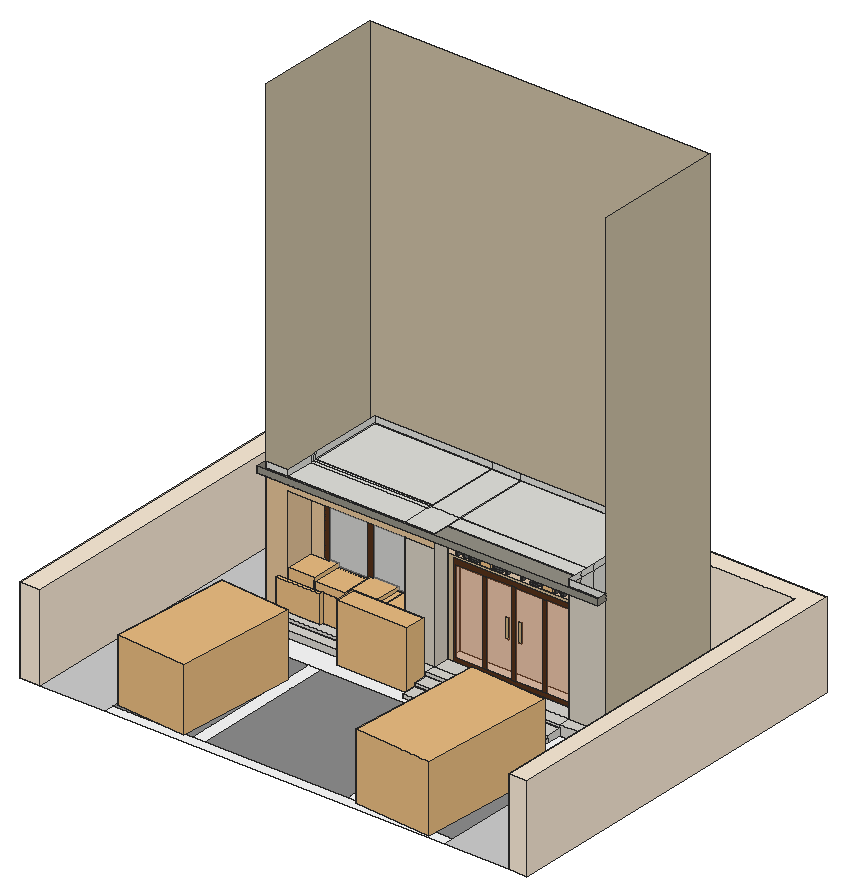
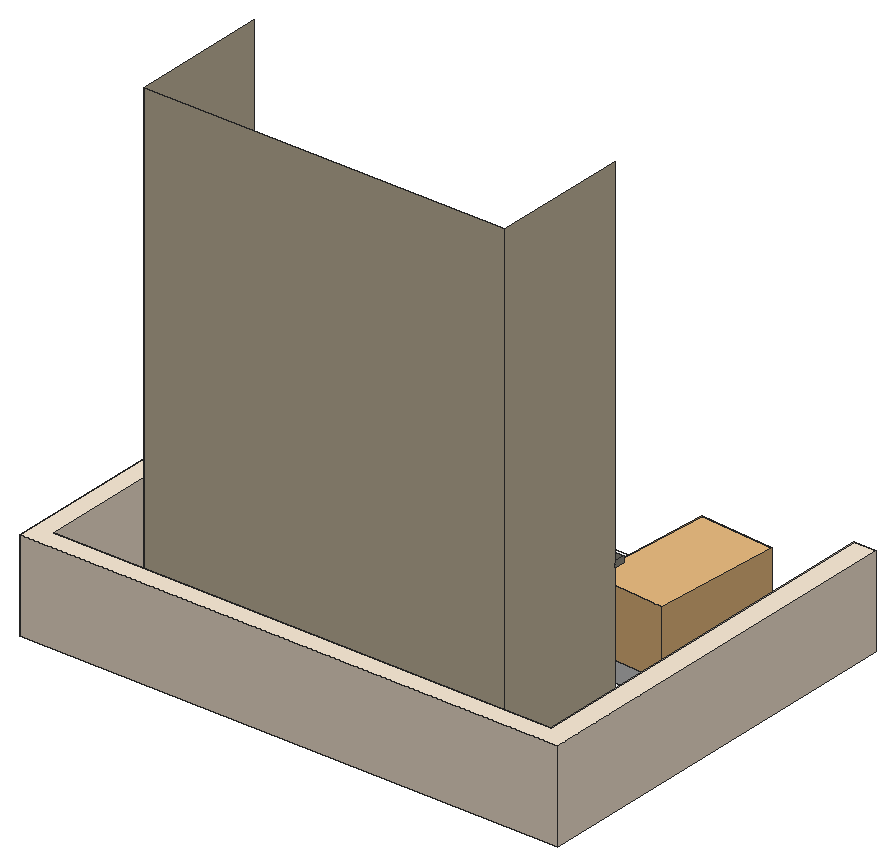
# SketchUp Ruby script. Lengths in inches.
U = 1.inch
M = Sketchup.active_model
def pt(a) = Geom::Point3d.new(a.map { |v| v * U })
def face(e, loops, mat)
  f = e.add_face(loops[0].map { |a| pt(a) })
  loops[1..].each { |l| e.add_face(l.map { |a| pt(a) }).erase! }
  f.material = f.back_material = mat if mat
  f
end
# faces: each face lists its corners as indices into pts; further lists are holes
def faces(e, pts, list, mat = nil) = list.each { |f| face(e, (f[0].is_a?(Array) ? f : [f]).map { |l| l.map { |i| pts[i] } }, mat) }
# xy, xz, yz: faces in a plane at the given z, y or x. An outline is a flat list of corners, or four numbers for a rectangle; further outlines are holes
def ring(l) = l.size == 4 ? [[l[0], l[1]], [l[2], l[1]], [l[2], l[3]], [l[0], l[3]]] : l.each_slice(2).to_a
def flat(e, list, mat, &to3) = list.each { |f| face(e, (f[0].is_a?(Array) ? f : [f]).map { |l| ring(l).map { |u, v| to3.(u, v) } }, mat) }
def xy(e, z, list, mat = nil) = flat(e, list, mat) { |x, y| [x, y, z] }
def xz(e, y, list, mat = nil) = flat(e, list, mat) { |x, z| [x, y, z] }
def yz(e, x, list, mat = nil) = flat(e, list, mat) { |y, z| [x, y, z] }
def lines(e, pts, list) = list.each { |a, b| e.add_line(pt(pts[a]), pt(pts[b])) }
# prism: a flat outline (further loops are holes) pulled along v
def prism(e, loops, v, mat = nil)
  f = face(e, loops, mat); d = Geom::Vector3d.new(v.map { |x| x * U })
  f.pushpull(f.normal.samedirection?(d) ? d.length : -d.length)
end
def box(e, o, s, mat = nil) = prism(e, [[o, [o[0] + s[0], o[1], o[2]], [o[0] + s[0], o[1] + s[1], o[2]], [o[0], o[1] + s[1], o[2]]]], [0, 0, s[2]], mat)
def at(x, y, z, deg = 0) = Geom::Transformation.translation(pt([x, y, z])) * Geom::Transformation.rotation(ORIGIN, Z_AXIS, deg.degrees)
def axes(o, x, y, z) = Geom::Transformation.new([*x, 0, *y, 0, *z, 0, *pt(o).to_a, 1])
def part(name) = M.definitions.add(name)
# library, detail: a bought-in or finely detailed component or shape, given as its bounding box
def library(name, o, s) = part(name).tap { |d| box(d.entities, o, s) }
def detail(e, o, s) = box(e.add_group.entities, o, s)
def put(e, d, t, mat = nil) = e.add_instance(d, t).tap { |i| i.material = mat if mat }
def group(e, t, mat = nil) = e.add_group.tap { |g| g.transformation = t; g.material = mat if mat }.entities
root = M.entities
M.materials.add("[0028_AntiqueWhite]").color = [250, 235, 215]
M.materials.add("[0035_Tan]").color = [229, 196, 153]
M.materials.add("[Carrera Marble]").color = [207, 207, 207]
M.materials.add("[Cinder Block]").color = [216, 208, 194]
M.materials.add("[Color M00]").color = [255, 255, 255]
M.materials.add("[Color M04]").color = [142, 142, 142]
M.materials.add("[Color M06]").color = [86, 86, 86]
M.materials.add("[Concrete Tile]").color = [203, 190, 164]
M.materials.add("[Formica Beige]").color = [211, 187, 149]
M.materials.add("[Formica Graystone]").color = [149, 146, 135]
M.materials.add("[Formica Laminate Light]").color = [255, 226, 196]
M.materials.add("[Terrazzo Tile Light]").color = [219, 217, 210]
M.materials.add("[Translucent Glass Gray]1").color = [193, 193, 193]
M.materials["[Translucent Glass Gray]1"].alpha = 0.5
M.materials.add("[Translucent Glass Gray]2").color = [249, 125, 51]
M.materials["[Translucent Glass Gray]2"].alpha = 0.31
M.materials.add("[Wood Floor Light]").color = [204, 176, 127]
M.materials.add("[Wood Veneer 01]").color = [86, 50, 26]
c1 = library("2015 Porsche Macan",[0.14,0.6,0.32],[90.05,184.43,65.58])
c2 = library("skpE847",[-111.76,-15.01,0.76],[2.12,4.6,1.82])
c3 = part("car+1")
p = [[0,0,0],[1,0,0],[1,1,0]]
lines(c3.entities,p,[[0,1],[1,2],[2,0]])
put(c3.entities,c2,axes([-477.97,5140.8,-31.25],[0,46,0],[-46,0,0],[0,0,40.94]))
c4 = library("Sem+nome",[-20.92,-6.25,0],[92.79,42.83,52.11])
c5 = library("chau cay",[-24.34,-109.24,0],[56.46,62.58,79.69])
c6 = library("Flora+17",[-57.52,158.6,-38.64],[66.99,62.88,77.28])
c7 = part("RECEPTION\#1")
prism(c7.entities,[[[4.13,0.7,0],[4.13,29.49,0],[12.1875,29.49,0],[16.45,29.28,0],[19.17,28.66,0],[20.99,27.63,0],[22.3,26.27,0],[23.08,24.58,0],[23.34,22.56,0],[22.98,19.8,0],[21.89,17.54,0],[19.96,15.6,0],[17.05,13.8,0],[26.99,0.7,0],[21.64,0.7,0],[12.55,12.68,0],[8.55,12.68,0],[8.55,0.7,0]],[[8.55,16,0],[10.89,16,0],[14.08,16.4,0],[16.54,17.58,0],[17.45,18.43,0],[18.11,19.43,0],[18.5,20.56,0],[18.63,21.83,0],[18.24,23.93,0],[17.74,24.6875,0],[17.06,25.25,0],[14.82,25.9375,0],[11.27,26.17,0],[8.55,26.17,0]]],[0,0,12])
prism(c7.entities,[[[32.54,0.7,0],[32.54,29.49,0],[52,29.49,0],[52,26.17,0],[36.97,26.17,0],[36.97,17.4375,0],[49.71,17.4375,0],[49.71,14.12,0],[36.97,14.12,0],[36.97,4.02,0],[53.03,4.02,0],[53.03,0.7,0]]],[0,0,12])
prism(c7.entities,[[[87.94,0.7,0],[87.94,29.49,0],[107.39,29.49,0],[107.39,26.17,0],[92.36,26.17,0],[92.36,17.4375,0],[105.1,17.4375,0],[105.1,14.12,0],[92.36,14.12,0],[92.36,4.02,0],[108.43,4.02,0],[108.43,0.7,0]]],[0,0,12])
prism(c7.entities,[[[115.9,0.7,0],[115.9,29.49,0],[125.27,29.49,0],[129.5625,29.27,0],[132.41,28.59,0],[134.32,27.43,0],[135.68,25.83,0],[136.5,23.8,0],[136.77,21.32,0],[136.55,19.18,0],[135.89,17.28,0],[134.79,15.62,0],[133.26,14.21,0],[131.33,13.08,0],[129.07,12.27,0],[126.48,11.79,0],[123.56,11.625,0],[120.32,11.625,0],[120.32,0.7,0]],[[120.32,14.95,0],[123.08,14.95,0],[127.01,15.34,0],[128.55,15.83,0],[129.82,16.52,0],[130.8,17.4,0],[131.5,18.48,0],[131.92,19.76,0],[132.06,21.23,0],[131.64,23.5,0],[131.11,24.36,0],[130.37,25.02,0],[128.11,25.88,0],[124.72,26.17,0],[120.32,26.17,0]]],[0,0,12])
prism(c7.entities,[[[150.1,0.7,0],[150.1,26.17,0],[139.04,26.17,0],[139.04,29.49,0],[165.61,29.49,0],[165.61,26.17,0],[154.53,26.17,0],[154.53,0.7,0]]],[0,0,12])
prism(c7.entities,[[[170.06,0.7,0],[170.06,4.02,0],[177.8,4.02,0],[177.8,26.17,0],[170.06,26.17,0],[170.06,29.49,0],[189.97,29.49,0],[189.97,26.17,0],[182.22,26.17,0],[182.22,4.02,0],[189.97,4.02,0],[189.97,0.7,0]]],[0,0,12])
prism(c7.entities,[[[224.89,0.7,0],[224.89,29.58,0],[229.08,29.58,0],[242.28,8.66,0],[242.33,8.66,0],[242.33,29.58,0],[245.94,29.58,0],[245.94,0.7,0],[241.86,0.7,0],[228.57,21.8125,0],[228.5,21.8125,0],[228.5,0.7,0]]],[0,0,12])
detail(c7.entities,[57.68,0,0],[23.63,30.1875,12])
detail(c7.entities,[195.26,0,0],[24.94,30.1875,12])
xy(root,0,[[0,0,0,788.125,1065.8,788.125,1065.8,0,1027.95,0,1027.95,751.09,42.72,751.09,42.72,0],[532.75,339.96,814,370.87],[532.75,370.87,814,401.78],[177.7,378.62,470.31,401.78],[177.7,401.78,893.35,697.17]])
xy(root,0,[[42.72,0,42.72,751.09,1027.95,751.09,1027.95,0,893.35,0,893.35,697.17,177.7,697.17,177.7,0]],"[Carrera Marble]")
xy(root,0,[[177.7,0,893.35,22.32],[344.92,22.32,370.54,328.57],[671.29,22.32,696.92,328.57],[177.7,328.57,177.7,378.62,470.31,378.62,470.31,401.78,532.75,401.78,532.75,339.96,814,339.96,814,401.78,893.35,401.78,893.35,328.57]],"[Color M00]")
xy(root,0,[[177.7,22.32,344.92,328.57],[370.54,22.32,671.29,328.57],[696.92,22.32,893.35,328.57]],"[Color M04]")
xy(root,8,[[532.75,339.96,814,370.87]],"[Terrazzo Tile Light]")
xy(root,13.875,[[177.7,378.62,470.31,401.78]],"[Terrazzo Tile Light]")
xy(root,14.125,[[532.75,370.87,814,401.78]],"[Terrazzo Tile Light]")
xy(root,21.25,[[470.31,423.82,532.75,651.39],[532.75,457.36,814,490.9],[231.36,482.68,470.31,496.86],[532.75,490.9,814,651.39],[225.05,496.86,470.31,651.39]])
xy(root,21.25,[[177.7,401.78,470.31,423.82],[470.31,401.78,532.75,423.82],[532.75,401.78,814,423.82],[814,401.78,893.35,423.82],[225.05,423.82,470.31,482.68],
  [532.75,423.82,814,457.36]],"[Terrazzo Tile Light]")
xy(root,180.0625,[[0,0,42.72,0,42.72,751.09,1027.95,751.09,1027.95,0,1065.8,0,1065.8,788.125,0,788.125]],"[0028_AntiqueWhite]")
xy(root,244.23,[[225.05,423.82,470.31,482.68]],"[Formica Beige]")
xy(root,272.25,[[225.05,423.82,470.31,482.68],[470.31,423.82,532.75,490.9],[532.75,457.36,814,490.9],[225.05,482.68,231.36,490.9],[231.36,482.68,470.31,490.9],
  [225.05,490.9,231.36,496.86],[231.36,490.9,470.31,496.86],[470.31,490.9,532.75,651.39],[532.75,490.9,814,651.39],[225.05,496.86,470.31,651.39]])
xy(root,272.25,[[177.7,401.69,470.31,423.82],[470.31,401.69,532.75,423.82],[532.75,401.69,532.75,457.36,814,457.36,814,423.82,893.35,423.82,893.35,401.69]],"[Formica Graystone]")
xz(root,0,[[0,0,42.72,180.0625],[1027.95,0,1065.8,180.0625]],"[0028_AntiqueWhite]")
xz(root,339.96,[[532.75,0,814,8]],"[Terrazzo Tile Light]")
xz(root,370.87,[[532.75,0,814,8]])
xz(root,370.87,[[532.75,8,814,14.125]],"[Terrazzo Tile Light]")
xz(root,378.62,[[177.7,0,470.31,13.875]],"[Terrazzo Tile Light]")
xz(root,401.69,[[177.7,272.25,893.35,285.1875]],"[Formica Graystone]")
xz(root,401.78,[[177.7,0,470.31,13.875],[532.75,0,814,14.125]])
xz(root,401.78,[[470.31,0,532.75,21.25],[814,0,893.35,21.25],[177.7,13.875,470.31,21.25],[532.75,14.125,814,21.25]],"[Terrazzo Tile Light]")
xz(root,423.82,[[177.7,272.25,225.05,285.1875],[814,272.25,893.35,285.1875]])
xz(root,423.82,[[177.7,21.25,225.05,21.25,225.05,244.23,532.75,244.23,532.75,272.25,177.7,272.25]],"[0035_Tan]")
xz(root,423.82,[[470.31,21.25,532.75,244.23],[814,21.25,893.35,272.25]],"[Cinder Block]")
xz(root,457.36,[[532.75,21.25,543.3,21.25,543.3,216.95,802.99,216.95,802.99,21.25,814,21.25,814,221.58,532.75,221.58]],"[Formica Beige]")
xz(root,457.36,[[532.75,221.58,814,272.25]],"[Formica Laminate Light]")
xz(root,457.36,[[551.32,29.27,606.59,205.95],[[615.14,29.27,668.4,205.95],[656.6875,104.04,662.8125,144.35]],[[676.95,29.27,733.65,205.95],[682.4375,104.04,688.5625,144.35]],[742.2,29.27,794.97,205.95]],"[Translucent Glass Gray]2")
xz(root,457.36,[[656.6875,104.04,662.8125,144.35],[682.4375,104.04,688.5625,144.35]],"[Wood Floor Light]")
xz(root,457.36,[[[543.3,21.25,802.99,216.95],[551.32,29.27,794.97,205.95]],[606.59,29.27,615.14,205.95],[668.4,29.27,676.95,205.95],[733.65,29.27,742.2,205.95]],"[Wood Veneer 01]")
xz(root,482.68,[[[225.05,21.25,470.31,244.23],[254.5,83.63,445.63,223.63]]],"[0035_Tan]")
xz(root,482.68,[[265.36,94.49,345.43,212.77],[357.18,94.49,434.77,212.77]],"[Translucent Glass Gray]1")
xz(root,482.68,[[[254.5,83.63,445.63,223.63],[265.36,94.49,434.77,212.77]],[345.43,94.49,357.18,212.77]],"[Wood Veneer 01]")
xz(root,490.9,[[532.75,21.25,814,272.25]])
xz(root,496.86,[[225.05,21.25,231.36,272.25],[231.36,21.25,470.31,272.25]])
xz(root,651.39,[[225.05,21.25,470.31,272.25],[470.31,21.25,532.75,272.25],[532.75,21.25,814,272.25],[225.05,272.25,470.31,285.1875],[470.31,272.25,532.75,285.1875],
  [532.75,272.25,814,285.1875]])
xz(root,697.17,[[177.7,0,893.35,994.25]],"[Concrete Tile]")
xz(root,751.09,[[42.72,0,1027.95,180.0625]],"[0028_AntiqueWhite]")
xz(root,788.125,[[0,0,1065.8,180.0625]],"[0028_AntiqueWhite]")
yz(root,0,[[0,0,788.125,180.0625]],"[0028_AntiqueWhite]")
yz(root,42.72,[[0,0,751.09,180.0625]],"[0028_AntiqueWhite]")
yz(root,177.7,[[401.78,0,401.78,21.25,423.82,21.25,423.82,994.25,697.17,994.25,697.17,0]],"[Concrete Tile]")
yz(root,177.7,[[401.69,272.25,423.82,285.1875]],"[Formica Graystone]")
yz(root,177.7,[[378.62,0,401.78,13.875]],"[Terrazzo Tile Light]")
yz(root,225.05,[[496.86,21.25,651.39,272.25],[423.82,272.25,482.68,285.1875],[482.68,272.25,490.9,285.1875],[490.9,272.25,496.86,285.1875],[496.86,272.25,651.39,285.1875]])
yz(root,225.05,[[423.82,21.25,482.68,244.23]],"[0035_Tan]")
yz(root,470.31,[[482.68,21.25,496.86,272.25],[496.86,21.25,651.39,272.25]])
yz(root,470.31,[[423.82,21.25,482.68,244.23]],"[0035_Tan]")
yz(root,470.31,[[378.62,0,401.78,13.875]],"[Terrazzo Tile Light]")
yz(root,532.75,[[457.36,21.25,490.9,272.25],[490.9,21.25,651.39,272.25]])
yz(root,532.75,[[423.82,21.25,457.36,272.25]],"[Cinder Block]")
yz(root,532.75,[[339.96,0,370.87,8],[370.87,0,401.78,14.125]],"[Terrazzo Tile Light]")
yz(root,814,[[457.36,21.25,490.9,272.25],[490.9,21.25,651.39,272.25],[423.82,272.25,457.36,285.1875],[457.36,272.25,490.9,285.1875],[490.9,272.25,651.39,285.1875]])
yz(root,814,[[423.82,21.25,457.36,272.25]],"[Cinder Block]")
yz(root,814,[[339.96,0,370.87,8],[370.87,0,401.78,14.125]],"[Terrazzo Tile Light]")
yz(root,893.35,[[401.78,0,697.17,0,697.17,994.25,423.82,994.25,423.82,21.25,401.78,21.25]],"[Concrete Tile]")
yz(root,893.35,[[401.69,272.25,423.82,285.1875]],"[Formica Graystone]")
yz(root,1027.95,[[0,0,751.09,180.0625]],"[0028_AntiqueWhite]")
yz(root,1065.8,[[0,0,788.125,180.0625]],"[0028_AntiqueWhite]")
put(root,c1,axes([873.99,289.53,-0.68],[-1.8043,0.11247,0],[-0.09564,-1.53422,0],[0,0,2.132]))
put(root,c3,axes([330.22,16.24,0],[0.08716,1.1868,0],[-1.51691,0.11141,0],[0,0,1.7792]))
put(root,c4,axes([413.51,363.66,0],[1.59657,0,0],[0,1,0],[0,0,2.34464]))
put(root,c4,axes([225.05,423.82,21.25],[1,0,0],[0,1,0],[0,0,1.10858]))
put(root,c5,at(249.39,533.06,21.25))
put(root,c5,at(450.375,533.06,21.25))
put(root,c6,axes([431.86,265.22,57.87],[0.9576,0,0],[0,1,0],[0,0,0.94765]))
put(root,c6,axes([334.24,265.22,57.87],[0.9576,0,0],[0,1,0],[0,0,0.94765]))
put(root,c4,axes([287.71,430.07,21.25],[1,0,0],[0,1,0],[0,0,1.10858]))
put(root,c5,at(374.89,533.06,21.25))
put(root,c7,axes([556.27,457.36,232.07],[0.9409,0,0],[0,0,0.94],[0,-1,0]),"[Color M06]")
